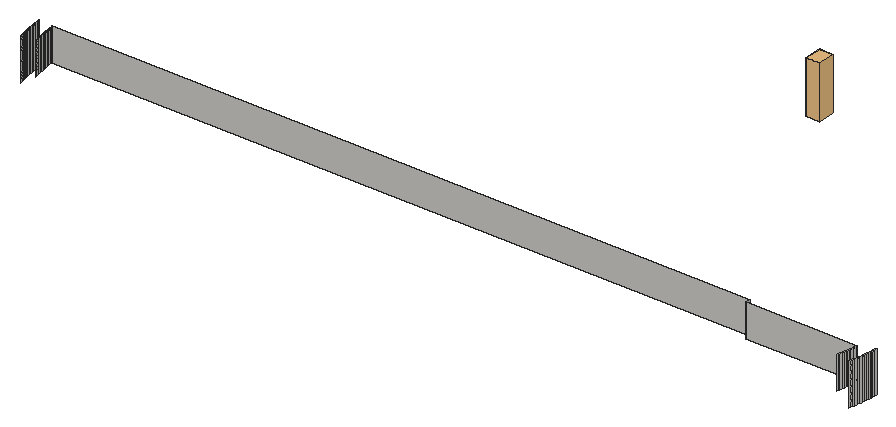
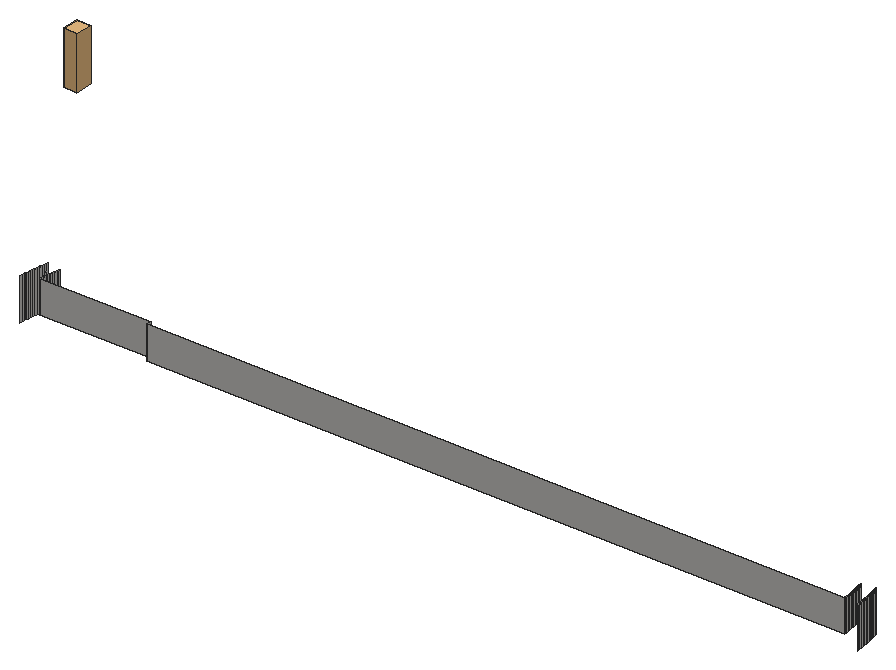
# SketchUp Ruby script. Lengths in inches.
U = 1.inch
M = Sketchup.active_model
def pt(a) = Geom::Point3d.new(a.map { |v| v * U })
def face(e, loops, mat)
  f = e.add_face(loops[0].map { |a| pt(a) })
  loops[1..].each { |l| e.add_face(l.map { |a| pt(a) }).erase! }
  f.material = f.back_material = mat if mat
  f
end
# faces: each face lists its corners as indices into pts; further lists are holes
def faces(e, pts, list, mat = nil) = list.each { |f| face(e, (f[0].is_a?(Array) ? f : [f]).map { |l| l.map { |i| pts[i] } }, mat) }
# xy, xz, yz: faces in a plane at the given z, y or x. An outline is a flat list of corners, or four numbers for a rectangle; further outlines are holes
def ring(l) = l.size == 4 ? [[l[0], l[1]], [l[2], l[1]], [l[2], l[3]], [l[0], l[3]]] : l.each_slice(2).to_a
def flat(e, list, mat, &to3) = list.each { |f| face(e, (f[0].is_a?(Array) ? f : [f]).map { |l| ring(l).map { |u, v| to3.(u, v) } }, mat) }
def xy(e, z, list, mat = nil) = flat(e, list, mat) { |x, y| [x, y, z] }
def xz(e, y, list, mat = nil) = flat(e, list, mat) { |x, z| [x, y, z] }
def yz(e, x, list, mat = nil) = flat(e, list, mat) { |y, z| [x, y, z] }
def lines(e, pts, list) = list.each { |a, b| e.add_line(pt(pts[a]), pt(pts[b])) }
# prism: a flat outline (further loops are holes) pulled along v
def prism(e, loops, v, mat = nil)
  f = face(e, loops, mat); d = Geom::Vector3d.new(v.map { |x| x * U })
  f.pushpull(f.normal.samedirection?(d) ? d.length : -d.length)
end
def box(e, o, s, mat = nil) = prism(e, [[o, [o[0] + s[0], o[1], o[2]], [o[0] + s[0], o[1] + s[1], o[2]], [o[0], o[1] + s[1], o[2]]]], [0, 0, s[2]], mat)
def at(x, y, z, deg = 0) = Geom::Transformation.translation(pt([x, y, z])) * Geom::Transformation.rotation(ORIGIN, Z_AXIS, deg.degrees)
def axes(o, x, y, z) = Geom::Transformation.new([*x, 0, *y, 0, *z, 0, *pt(o).to_a, 1])
def part(name) = M.definitions.add(name)
# library, detail: a bought-in or finely detailed component or shape, given as its bounding box
def library(name, o, s) = part(name).tap { |d| box(d.entities, o, s) }
def detail(e, o, s) = box(e.add_group.entities, o, s)
def put(e, d, t, mat = nil) = e.add_instance(d, t).tap { |i| i.material = mat if mat }
def group(e, t, mat = nil) = e.add_group.tap { |g| g.transformation = t; g.material = mat if mat }.entities
root = M.entities
M.materials.add("[Stone Sandstone Ashlar Light]").color = [201, 199, 196]
c1 = library("WALL LIGHT 69",[4.19,4.05,-9.07],[4.61,5.7,17.71])
xz(root,33,[[369,-10,392.79,-3]],"[Stone Sandstone Ashlar Light]")
xz(root,34,[[219.12,-10,369,-3]],"[Stone Sandstone Ashlar Light]")
yz(root,369,[[33,-10,34,-3]],"[Stone Sandstone Ashlar Light]")
p = [[216.98,28.13,-3],[216.9,28.51,-3],[216.9,28.51,-12],[216.98,28.13,-12],[395.1,28.51,-3],[395.02,28.13,-3],
  [395.02,28.13,-12],[395.1,28.51,-12],[216.82,28.89,-3],[216.82,28.89,-12],[395.18,28.89,-3],[395.18,28.89,-12],
  [216.74,29.28,-3],[216.74,29.28,-12],[395.26,29.28,-3],[395.26,29.28,-12],[216.67,29.66,-3],[216.67,29.66,-12],
  [395.33,29.66,-3],[395.33,29.66,-12],[216.6,30.04,-3],[216.6,30.04,-12],[395.4,30.04,-3],[395.4,30.04,-12],
  [216.54,30.42,-3],[216.54,30.42,-12],[395.46,30.42,-3],[395.46,30.42,-12],[216.48,30.81,-3],[216.48,30.81,-12],
  [395.52,30.81,-3],[395.52,30.81,-12],[216.42,31.19,-3],[216.42,31.19,-12],[395.58,31.19,-3],[395.58,31.19,-12],
  [216.36,31.58,-3],[216.36,31.58,-12],[395.64,31.58,-3],[395.64,31.58,-12],[216.31,31.96,-3],[216.31,31.96,-12],
  [395.69,31.96,-3],[395.69,31.96,-12],[216.27,32.35,-3],[216.27,32.35,-12],[395.73,32.35,-3],[395.73,32.35,-12],
  [216.23,32.73,-3],[216.23,32.73,-12],[395.77,32.73,-3],[395.77,32.73,-12],[216.1875,33.12,-3],[216.1875,33.12,-12],
  [395.8125,33.12,-3],[395.8125,33.12,-12],[216.15,33.51,-3],[216.15,33.51,-12],[395.85,33.51,-3],[395.85,33.51,-12],
  [216.12,33.89,-3],[216.12,33.89,-12],[395.88,33.89,-3],[395.88,33.89,-12],[216.09,34.28,-3],[216.09,34.28,-12],
  [395.91,34.28,-3],[395.91,34.28,-12],[219.91,28.79,-3],[219.99,28.44,-3],[219.99,28.44,-10],[219.91,28.79,-10],
  [392.01,28.44,-3],[392.09,28.79,-3],[392.09,28.79,-10],[392.01,28.44,-10],[219.83,29.14,-3],[219.83,29.14,-10],
  [392.17,29.14,-3],[392.17,29.14,-10],[219.76,29.49,-3],[219.76,29.49,-10],[392.24,29.49,-3],[392.24,29.49,-10],
  [219.6875,29.85,-3],[219.6875,29.85,-10],[392.3125,29.85,-3],[392.3125,29.85,-10],[219.62,30.2,-3],[219.62,30.2,-10],
  [392.38,30.2,-3],[392.38,30.2,-10],[219.56,30.56,-3],[219.56,30.56,-10],[392.44,30.56,-3],[392.44,30.56,-10],
  [219.5,30.91,-3],[219.5,30.91,-10],[392.5,30.91,-3],[392.5,30.91,-10],[219.44,31.27,-3],[219.44,31.27,-10],
  [392.56,31.27,-3],[392.56,31.27,-10],[219.39,31.62,-3],[219.39,31.62,-10],[392.61,31.62,-3],[392.61,31.62,-10],
  [219.34,31.98,-3],[219.34,31.98,-10],[392.66,31.98,-3],[392.66,31.98,-10],[219.29,32.33,-3],[219.29,32.33,-10],
  [392.71,32.33,-3],[392.71,32.33,-10],[219.25,32.69,-3],[219.25,32.69,-10],[392.75,32.69,-3],[392.75,32.69,-10],
  [219.21,33.05,-3],[219.21,33.05,-10],[392.79,33,-3],[392.79,33,-10],[219.17,33.41,-3],[219.17,33.41,-10],
  [219.14,33.77,-3],[219.14,33.77,-10],[219.12,34,-3],[219.12,34,-10]]
faces(root,p,[[0,1,2,3],[4,5,6,7],[1,8,9,2],[10,4,7,11],[8,12,13,9],[14,10,11,15],[12,16,17,13],[18,14,15,19],
  [16,20,21,17],[22,18,19,23],[20,24,25,21],[26,22,23,27],[24,28,29,25],[30,26,27,31],[28,32,33,29],[34,30,31,35],
  [32,36,37,33],[38,34,35,39],[36,40,41,37],[42,38,39,43],[40,44,45,41],[46,42,43,47],[44,48,49,45],[50,46,47,51],
  [48,52,53,49],[54,50,51,55],[52,56,57,53],[58,54,55,59],[56,60,61,57],[62,58,59,63],[60,64,65,61],[66,62,63,67],
  [68,69,70,71],[72,73,74,75],[76,68,71,77],[73,78,79,74],[80,76,77,81],[78,82,83,79],[84,80,81,85],[82,86,87,83],
  [88,84,85,89],[86,90,91,87],[92,88,89,93],[90,94,95,91],[96,92,93,97],[94,98,99,95],[100,96,97,101],[98,102,103,99],
  [104,100,101,105],[102,106,107,103],[108,104,105,109],[106,110,111,107],[112,108,109,113],[110,114,115,111],[116,112,113,117],[114,118,119,115],
  [120,116,117,121],[118,122,123,119],[124,120,121,125],[126,124,125,127],[128,126,127,129]],"[Stone Sandstone Ashlar Light]")
put(root,c1,axes([379.65,29.76,43.54],[0.64,0,0],[0,0.64,0],[0,0,0.64]))
